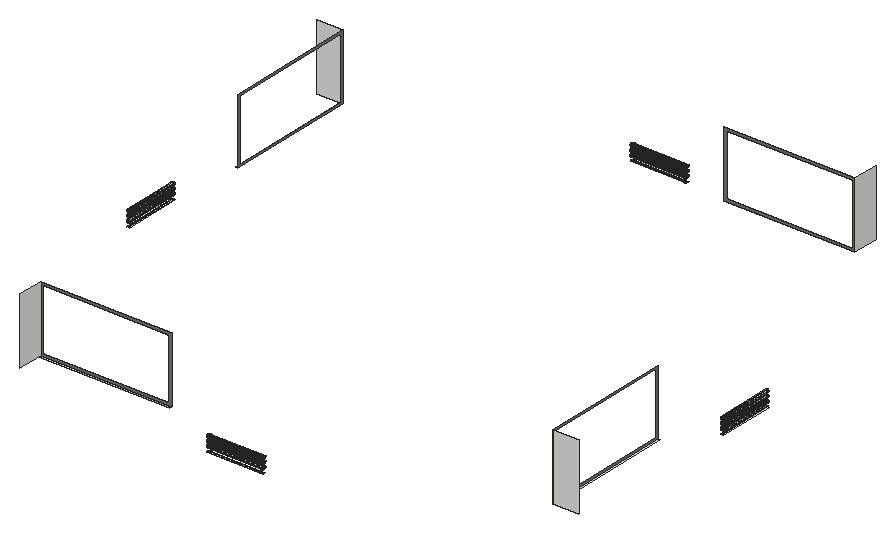
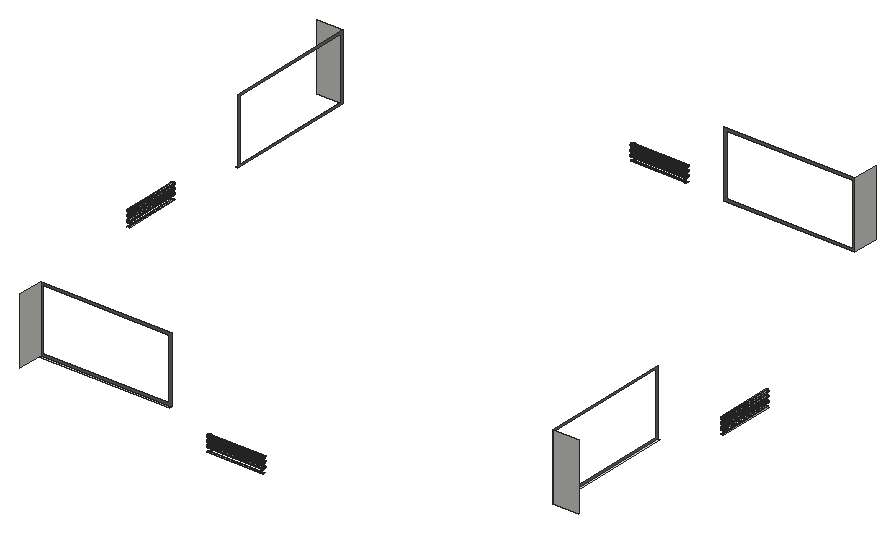
# SketchUp Ruby script. Lengths in inches.
U = 1.inch
M = Sketchup.active_model
def pt(a) = Geom::Point3d.new(a.map { |v| v * U })
def face(e, loops, mat)
  f = e.add_face(loops[0].map { |a| pt(a) })
  loops[1..].each { |l| e.add_face(l.map { |a| pt(a) }).erase! }
  f.material = f.back_material = mat if mat
  f
end
# faces: each face lists its corners as indices into pts; further lists are holes
def faces(e, pts, list, mat = nil) = list.each { |f| face(e, (f[0].is_a?(Array) ? f : [f]).map { |l| l.map { |i| pts[i] } }, mat) }
# xy, xz, yz: faces in a plane at the given z, y or x. An outline is a flat list of corners, or four numbers for a rectangle; further outlines are holes
def ring(l) = l.size == 4 ? [[l[0], l[1]], [l[2], l[1]], [l[2], l[3]], [l[0], l[3]]] : l.each_slice(2).to_a
def flat(e, list, mat, &to3) = list.each { |f| face(e, (f[0].is_a?(Array) ? f : [f]).map { |l| ring(l).map { |u, v| to3.(u, v) } }, mat) }
def xy(e, z, list, mat = nil) = flat(e, list, mat) { |x, y| [x, y, z] }
def xz(e, y, list, mat = nil) = flat(e, list, mat) { |x, z| [x, y, z] }
def yz(e, x, list, mat = nil) = flat(e, list, mat) { |y, z| [x, y, z] }
def lines(e, pts, list) = list.each { |a, b| e.add_line(pt(pts[a]), pt(pts[b])) }
# prism: a flat outline (further loops are holes) pulled along v
def prism(e, loops, v, mat = nil)
  f = face(e, loops, mat); d = Geom::Vector3d.new(v.map { |x| x * U })
  f.pushpull(f.normal.samedirection?(d) ? d.length : -d.length)
end
def box(e, o, s, mat = nil) = prism(e, [[o, [o[0] + s[0], o[1], o[2]], [o[0] + s[0], o[1] + s[1], o[2]], [o[0], o[1] + s[1], o[2]]]], [0, 0, s[2]], mat)
def at(x, y, z, deg = 0) = Geom::Transformation.translation(pt([x, y, z])) * Geom::Transformation.rotation(ORIGIN, Z_AXIS, deg.degrees)
def axes(o, x, y, z) = Geom::Transformation.new([*x, 0, *y, 0, *z, 0, *pt(o).to_a, 1])
def part(name) = M.definitions.add(name)
# library, detail: a bought-in or finely detailed component or shape, given as its bounding box
def library(name, o, s) = part(name).tap { |d| box(d.entities, o, s) }
def detail(e, o, s) = box(e.add_group.entities, o, s)
def put(e, d, t, mat = nil) = e.add_instance(d, t).tap { |i| i.material = mat if mat }
def group(e, t, mat = nil) = e.add_group.tap { |g| g.transformation = t; g.material = mat if mat }.entities
root = M.entities
M.materials.add("[Metal Seamed]").color = [118, 119, 115]
xy(root,893.76,[[306.65,96.8125,641.22,102.8125],[1482,271.47,1488,606.03],[132,943.59,138,1278.16],[978.78,1446.8125,1313.35,1452.8125]])
xz(root,102.8125,[[[306.65,893.76,641.22,1062.625],[312.65,899.76,635.22,1056.625]]],"[Metal Seamed]")
xz(root,271.47,[[1482,893.76,1548,1062.625]])
xz(root,1278.16,[[72,893.76,138,1062.625]])
xz(root,1446.8125,[[[978.78,893.76,1313.35,1062.625],[984.78,899.76,1307.35,1056.625]]],"[Metal Seamed]")
yz(root,138,[[[943.59,893.76,1278.16,1062.625],[949.59,899.76,1272.16,1056.625]]],"[Metal Seamed]")
yz(root,306.65,[[36.8125,893.76,102.8125,1062.625]])
yz(root,1313.35,[[1446.8125,893.76,1512.8125,1062.625]])
yz(root,1482,[[[271.47,893.76,606.03,1062.625],[277.47,899.76,600.03,1056.625]]],"[Metal Seamed]")
p = [[922.01,45.15,863.55],[922.01,45.73,864.3125],[778.64,45.73,864.3125],[778.64,45.15,863.55],[922.01,50.95,864.3125],[922.01,51.53,863.55],
  [778.64,51.53,863.55],[778.64,50.95,864.3125],[80.33,662.8,863.55],[80.92,662.8,864.3125],[80.92,806.17,864.3125],[80.33,806.17,863.55],
  [86.13,662.8,864.3125],[86.72,662.8,863.55],[86.72,806.17,863.55],[86.13,806.17,864.3125],[1533.87,886.83,864.3125],[1533.28,886.83,863.55],
  [1533.28,743.45,863.55],[1533.87,743.45,864.3125],[1539.67,886.83,863.55],[1539.08,886.83,864.3125],[1539.08,743.45,864.3125],[1539.67,743.45,863.55],
  [697.99,1498.68,864.3125],[697.99,1498.09,863.55],[841.36,1498.09,863.55],[841.36,1498.68,864.3125],[697.99,1504.48,863.55],[697.99,1503.89,864.3125],
  [841.36,1503.89,864.3125],[841.36,1504.48,863.55],[922.01,46.5,864.9],[778.64,46.5,864.9],[922.01,50.18,864.9],[778.64,50.18,864.9],
  [81.68,662.8,864.9],[81.68,806.17,864.9],[85.37,662.8,864.9],[85.37,806.17,864.9],[1534.63,886.83,864.9],[1534.63,743.45,864.9],
  [1538.32,886.83,864.9],[1538.32,743.45,864.9],[697.99,1499.44,864.9],[841.36,1499.44,864.9],[697.99,1503.13,864.9],[841.36,1503.13,864.9],
  [922.01,47.38,865.27],[778.64,47.38,865.27],[922.01,49.29,865.27],[778.64,49.29,865.27],[82.57,662.8,865.27],[82.57,806.17,865.27],
  [84.48,662.8,865.27],[84.48,806.17,865.27],[1535.52,886.83,865.27],[1535.52,743.45,865.27],[1537.43,886.83,865.27],[1537.43,743.45,865.27],
  [697.99,1500.33,865.27],[841.36,1500.33,865.27],[697.99,1502.24,865.27],[841.36,1502.24,865.27],[922.01,48.34,865.39],[778.64,48.34,865.39],
  [83.53,662.8,865.39],[83.53,806.17,865.39],[1536.47,886.83,865.39],[1536.47,743.45,865.39],[697.99,1501.28,865.39],[841.36,1501.28,865.39],
  [922.01,48.34,873.02],[922.01,47.38,873.14],[778.64,47.38,873.14],[778.64,48.34,873.02],[922.01,49.29,873.14],[778.64,49.29,873.14],
  [83.53,662.8,873.02],[82.57,662.8,873.14],[82.57,806.17,873.14],[83.53,806.17,873.02],[84.48,662.8,873.14],[84.48,806.17,873.14],
  [1535.52,886.83,873.14],[1536.47,886.83,873.02],[1536.47,743.45,873.02],[1535.52,743.45,873.14],[1537.43,886.83,873.14],[1537.43,743.45,873.14],
  [697.99,1500.33,873.14],[697.99,1501.28,873.02],[841.36,1501.28,873.02],[841.36,1500.33,873.14],[697.99,1502.24,873.14],[841.36,1502.24,873.14],
  [922.01,46.5,873.51],[778.64,46.5,873.51],[922.01,50.18,873.51],[778.64,50.18,873.51],[81.68,662.8,873.51],[81.68,806.17,873.51],
  [85.37,662.8,873.51],[85.37,806.17,873.51],[1534.63,886.83,873.51],[1534.63,743.45,873.51],[1538.32,886.83,873.51],[1538.32,743.45,873.51],
  [697.99,1499.44,873.51],[841.36,1499.44,873.51],[697.99,1503.13,873.51],[841.36,1503.13,873.51],[922.01,45.73,874.1],[778.64,45.73,874.1],
  [922.01,50.95,874.1],[778.64,50.95,874.1],[80.92,662.8,874.1],[80.92,806.17,874.1],[86.13,662.8,874.1],[86.13,806.17,874.1],
  [1533.87,886.83,874.1],[1533.87,743.45,874.1],[1539.08,886.83,874.1],[1539.08,743.45,874.1],[697.99,1498.68,874.1],[841.36,1498.68,874.1],
  [697.99,1503.89,874.1],[841.36,1503.89,874.1],[922.01,45.15,874.86],[778.64,45.15,874.86],[922.01,51.53,874.86],[778.64,51.53,874.86],
  [80.33,662.8,874.86],[80.33,806.17,874.86],[86.72,662.8,874.86],[86.72,806.17,874.86],[1533.28,886.83,874.86],[1533.28,743.45,874.86],
  [1539.67,886.83,874.86],[1539.67,743.45,874.86],[697.99,1498.09,874.86],[841.36,1498.09,874.86],[697.99,1504.48,874.86],[841.36,1504.48,874.86],
  [922.01,44.78,875.75],[778.64,44.78,875.75],[922.01,51.9,875.75],[778.64,51.9,875.75],[79.97,662.8,875.75],[79.97,806.17,875.75],
  [87.09,662.8,875.75],[87.09,806.17,875.75],[1532.91,886.83,875.75],[1532.91,743.45,875.75],[1540.03,886.83,875.75],[1540.03,743.45,875.75],
  [697.99,1497.72,875.75],[841.36,1497.72,875.75],[697.99,1504.85,875.75],[841.36,1504.85,875.75],[922.01,44.65,876.7],[778.64,44.65,876.7],
  [922.01,52.03,876.7],[778.64,52.03,876.7],[79.84,662.8,876.7],[79.84,806.17,876.7],[87.21,662.8,876.7],[87.21,806.17,876.7],
  [1532.79,886.83,876.7],[1532.79,743.45,876.7],[1540.16,886.83,876.7],[1540.16,743.45,876.7],[697.99,1497.6,876.7],[841.36,1497.6,876.7],
  [697.99,1504.97,876.7],[841.36,1504.97,876.7],[922.01,44.78,877.66],[778.64,44.78,877.66],[922.01,51.9,877.66],[778.64,51.9,877.66],
  [79.97,662.8,877.66],[79.97,806.17,877.66],[87.09,662.8,877.66],[87.09,806.17,877.66],[1532.91,886.83,877.66],[1532.91,743.45,877.66],
  [1540.03,886.83,877.66],[1540.03,743.45,877.66],[697.99,1497.72,877.66],[841.36,1497.72,877.66],[697.99,1504.85,877.66],[841.36,1504.85,877.66],
  [922.01,45.15,878.55],[778.64,45.15,878.55],[922.01,51.53,878.55],[778.64,51.53,878.55],[80.33,662.8,878.55],[80.33,806.17,878.55],
  [86.72,662.8,878.55],[86.72,806.17,878.55],[1533.28,886.83,878.55],[1533.28,743.45,878.55],[1539.67,886.83,878.55],[1539.67,743.45,878.55],
  [697.99,1498.09,878.55],[841.36,1498.09,878.55],[697.99,1504.48,878.55],[841.36,1504.48,878.55],[922.01,45.73,879.3125],[778.64,45.73,879.3125],
  [922.01,50.95,879.3125],[778.64,50.95,879.3125],[80.92,662.8,879.3125],[80.92,806.17,879.3125],[86.13,662.8,879.3125],[86.13,806.17,879.3125],
  [1533.87,886.83,879.3125],[1533.87,743.45,879.3125],[1539.08,886.83,879.3125],[1539.08,743.45,879.3125],[697.99,1498.68,879.3125],[841.36,1498.68,879.3125],
  [697.99,1503.89,879.3125],[841.36,1503.89,879.3125],[922.01,46.5,879.9],[778.64,46.5,879.9],[922.01,50.18,879.9],[778.64,50.18,879.9],
  [81.68,662.8,879.9],[81.68,806.17,879.9],[85.37,662.8,879.9],[85.37,806.17,879.9],[1534.63,886.83,879.9],[1534.63,743.45,879.9],
  [1538.32,886.83,879.9],[1538.32,743.45,879.9],[697.99,1499.44,879.9],[841.36,1499.44,879.9],[697.99,1503.13,879.9],[841.36,1503.13,879.9],
  [922.01,47.38,880.27],[778.64,47.38,880.27],[922.01,49.29,880.27],[778.64,49.29,880.27],[82.57,662.8,880.27],[82.57,806.17,880.27],
  [84.48,662.8,880.27],[84.48,806.17,880.27],[1535.52,886.83,880.27],[1535.52,743.45,880.27],[1537.43,886.83,880.27],[1537.43,743.45,880.27],
  [697.99,1500.33,880.27],[841.36,1500.33,880.27],[697.99,1502.24,880.27],[841.36,1502.24,880.27],[922.01,48.34,880.39],[778.64,48.34,880.39],
  [83.53,662.8,880.39],[83.53,806.17,880.39],[1536.47,886.83,880.39],[1536.47,743.45,880.39],[697.99,1501.28,880.39],[841.36,1501.28,880.39],
  [922.01,48.34,885.02],[922.01,47.38,885.14],[778.64,47.38,885.14],[778.64,48.34,885.02],[922.01,49.29,885.14],[778.64,49.29,885.14],
  [83.53,662.8,885.02],[82.57,662.8,885.14],[82.57,806.17,885.14],[83.53,806.17,885.02],[84.48,662.8,885.14],[84.48,806.17,885.14],
  [1535.52,886.83,885.14],[1536.47,886.83,885.02],[1536.47,743.45,885.02],[1535.52,743.45,885.14],[1537.43,886.83,885.14],[1537.43,743.45,885.14],
  [697.99,1500.33,885.14],[697.99,1501.28,885.02],[841.36,1501.28,885.02],[841.36,1500.33,885.14],[697.99,1502.24,885.14],[841.36,1502.24,885.14],
  [922.01,46.5,885.51],[778.64,46.5,885.51],[922.01,50.18,885.51],[778.64,50.18,885.51],[81.68,662.8,885.51],[81.68,806.17,885.51],
  [85.37,662.8,885.51],[85.37,806.17,885.51],[1534.63,886.83,885.51],[1534.63,743.45,885.51],[1538.32,886.83,885.51],[1538.32,743.45,885.51],
  [697.99,1499.44,885.51],[841.36,1499.44,885.51],[697.99,1503.13,885.51],[841.36,1503.13,885.51],[922.01,45.73,886.1],[778.64,45.73,886.1],
  [922.01,50.95,886.1],[778.64,50.95,886.1],[80.92,662.8,886.1],[80.92,806.17,886.1],[86.13,662.8,886.1],[86.13,806.17,886.1],
  [1533.87,886.83,886.1],[1533.87,743.45,886.1],[1539.08,886.83,886.1],[1539.08,743.45,886.1],[697.99,1498.68,886.1],[841.36,1498.68,886.1],
  [697.99,1503.89,886.1],[841.36,1503.89,886.1],[922.01,45.15,886.86],[778.64,45.15,886.86],[922.01,51.53,886.86],[778.64,51.53,886.86],
  [80.33,662.8,886.86],[80.33,806.17,886.86],[86.72,662.8,886.86],[86.72,806.17,886.86],[1533.28,886.83,886.86],[1533.28,743.45,886.86],
  [1539.67,886.83,886.86],[1539.67,743.45,886.86],[697.99,1498.09,886.86],[841.36,1498.09,886.86],[697.99,1504.48,886.86],[841.36,1504.48,886.86],
  [922.01,44.78,887.75],[778.64,44.78,887.75],[922.01,51.9,887.75],[778.64,51.9,887.75],[79.97,662.8,887.75],[79.97,806.17,887.75],
  [87.09,662.8,887.75],[87.09,806.17,887.75],[1532.91,886.83,887.75],[1532.91,743.45,887.75],[1540.03,886.83,887.75],[1540.03,743.45,887.75],
  [697.99,1497.72,887.75],[841.36,1497.72,887.75],[697.99,1504.85,887.75],[841.36,1504.85,887.75],[922.01,44.65,888.7],[778.64,44.65,888.7],
  [922.01,52.03,888.7],[778.64,52.03,888.7],[79.84,662.8,888.7],[79.84,806.17,888.7],[87.21,662.8,888.7],[87.21,806.17,888.7],
  [1532.79,886.83,888.7],[1532.79,743.45,888.7],[1540.16,886.83,888.7],[1540.16,743.45,888.7],[697.99,1497.6,888.7],[841.36,1497.6,888.7],
  [697.99,1504.97,888.7],[841.36,1504.97,888.7],[922.01,44.78,889.66],[778.64,44.78,889.66],[922.01,51.9,889.66],[778.64,51.9,889.66],
  [79.97,662.8,889.66],[79.97,806.17,889.66],[87.09,662.8,889.66],[87.09,806.17,889.66],[1532.91,886.83,889.66],[1532.91,743.45,889.66],
  [1540.03,886.83,889.66],[1540.03,743.45,889.66],[697.99,1497.72,889.66],[841.36,1497.72,889.66],[697.99,1504.85,889.66],[841.36,1504.85,889.66],
  [922.01,45.15,890.55],[778.64,45.15,890.55],[922.01,51.53,890.55],[778.64,51.53,890.55],[80.33,662.8,890.55],[80.33,806.17,890.55],
  [86.72,662.8,890.55],[86.72,806.17,890.55],[1533.28,886.83,890.55],[1533.28,743.45,890.55],[1539.67,886.83,890.55],[1539.67,743.45,890.55],
  [697.99,1498.09,890.55],[841.36,1498.09,890.55],[697.99,1504.48,890.55],[841.36,1504.48,890.55],[922.01,45.73,891.3125],[778.64,45.73,891.3125],
  [922.01,50.95,891.3125],[778.64,50.95,891.3125],[80.92,662.8,891.3125],[80.92,806.17,891.3125],[86.13,662.8,891.3125],[86.13,806.17,891.3125],
  [1533.87,886.83,891.3125],[1533.87,743.45,891.3125],[1539.08,886.83,891.3125],[1539.08,743.45,891.3125],[697.99,1498.68,891.3125],[841.36,1498.68,891.3125],
  [697.99,1503.89,891.3125],[841.36,1503.89,891.3125],[922.01,46.5,891.9],[778.64,46.5,891.9],[922.01,50.18,891.9],[778.64,50.18,891.9],
  [81.68,662.8,891.9],[81.68,806.17,891.9],[85.37,662.8,891.9],[85.37,806.17,891.9],[1534.63,886.83,891.9],[1534.63,743.45,891.9],
  [1538.32,886.83,891.9],[1538.32,743.45,891.9],[697.99,1499.44,891.9],[841.36,1499.44,891.9],[697.99,1503.13,891.9],[841.36,1503.13,891.9],
  [922.01,47.38,892.27],[778.64,47.38,892.27],[922.01,49.29,892.27],[778.64,49.29,892.27],[82.57,662.8,892.27],[82.57,806.17,892.27],
  [84.48,662.8,892.27],[84.48,806.17,892.27],[1535.52,886.83,892.27],[1535.52,743.45,892.27],[1537.43,886.83,892.27],[1537.43,743.45,892.27],
  [697.99,1500.33,892.27],[841.36,1500.33,892.27],[697.99,1502.24,892.27],[841.36,1502.24,892.27],[922.01,48.34,892.39],[778.64,48.34,892.39],
  [83.53,662.8,892.39],[83.53,806.17,892.39],[1536.47,886.83,892.39],[1536.47,743.45,892.39],[697.99,1501.28,892.39],[841.36,1501.28,892.39],
  [922.01,48.34,897.02],[922.01,47.38,897.14],[778.64,47.38,897.14],[778.64,48.34,897.02],[922.01,49.29,897.14],[778.64,49.29,897.14],
  [83.53,662.8,897.02],[82.57,662.8,897.14],[82.57,806.17,897.14],[83.53,806.17,897.02],[84.48,662.8,897.14],[84.48,806.17,897.14],
  [1535.52,886.83,897.14],[1536.47,886.83,897.02],[1536.47,743.45,897.02],[1535.52,743.45,897.14],[1537.43,886.83,897.14],[1537.43,743.45,897.14],
  [697.99,1500.33,897.14],[697.99,1501.28,897.02],[841.36,1501.28,897.02],[841.36,1500.33,897.14],[697.99,1502.24,897.14],[841.36,1502.24,897.14],
  [922.01,46.5,897.51],[778.64,46.5,897.51],[922.01,50.18,897.51],[778.64,50.18,897.51],[81.68,662.8,897.51],[81.68,806.17,897.51],
  [85.37,662.8,897.51],[85.37,806.17,897.51],[1534.63,886.83,897.51],[1534.63,743.45,897.51],[1538.32,886.83,897.51],[1538.32,743.45,897.51],
  [697.99,1499.44,897.51],[841.36,1499.44,897.51],[697.99,1503.13,897.51],[841.36,1503.13,897.51],[922.01,45.73,898.1],[778.64,45.73,898.1],
  [922.01,50.95,898.1],[778.64,50.95,898.1],[80.92,662.8,898.1],[80.92,806.17,898.1],[86.13,662.8,898.1],[86.13,806.17,898.1],
  [1533.87,886.83,898.1],[1533.87,743.45,898.1],[1539.08,886.83,898.1],[1539.08,743.45,898.1],[697.99,1498.68,898.1],[841.36,1498.68,898.1],
  [697.99,1503.89,898.1],[841.36,1503.89,898.1],[922.01,45.15,898.86],[778.64,45.15,898.86],[922.01,51.53,898.86],[778.64,51.53,898.86],
  [80.33,662.8,898.86],[80.33,806.17,898.86],[86.72,662.8,898.86],[86.72,806.17,898.86],[1533.28,886.83,898.86],[1533.28,743.45,898.86],
  [1539.67,886.83,898.86],[1539.67,743.45,898.86],[697.99,1498.09,898.86],[841.36,1498.09,898.86],[697.99,1504.48,898.86],[841.36,1504.48,898.86],
  [922.01,44.78,899.75],[778.64,44.78,899.75],[922.01,51.9,899.75],[778.64,51.9,899.75],[79.97,662.8,899.75],[79.97,806.17,899.75],
  [87.09,662.8,899.75],[87.09,806.17,899.75],[1532.91,886.83,899.75],[1532.91,743.45,899.75],[1540.03,886.83,899.75],[1540.03,743.45,899.75],
  [697.99,1497.72,899.75],[841.36,1497.72,899.75],[697.99,1504.85,899.75],[841.36,1504.85,899.75],[922.01,44.65,900.7],[778.64,44.65,900.7],
  [922.01,52.03,900.7],[778.64,52.03,900.7],[79.84,662.8,900.7],[79.84,806.17,900.7],[87.21,662.8,900.7],[87.21,806.17,900.7],
  [1532.79,886.83,900.7],[1532.79,743.45,900.7],[1540.16,886.83,900.7],[1540.16,743.45,900.7],[697.99,1497.6,900.7],[841.36,1497.6,900.7],
  [697.99,1504.97,900.7],[841.36,1504.97,900.7],[922.01,44.78,901.66],[778.64,44.78,901.66],[922.01,51.9,901.66],[778.64,51.9,901.66],
  [79.97,662.8,901.66],[79.97,806.17,901.66],[87.09,662.8,901.66],[87.09,806.17,901.66],[1532.91,886.83,901.66],[1532.91,743.45,901.66],
  [1540.03,886.83,901.66],[1540.03,743.45,901.66],[697.99,1497.72,901.66],[841.36,1497.72,901.66],[697.99,1504.85,901.66],[841.36,1504.85,901.66],
  [922.01,45.15,902.55],[778.64,45.15,902.55],[922.01,51.53,902.55],[778.64,51.53,902.55],[80.33,662.8,902.55],[80.33,806.17,902.55],
  [86.72,662.8,902.55],[86.72,806.17,902.55],[1533.28,886.83,902.55],[1533.28,743.45,902.55],[1539.67,886.83,902.55],[1539.67,743.45,902.55],
  [697.99,1498.09,902.55],[841.36,1498.09,902.55],[697.99,1504.48,902.55],[841.36,1504.48,902.55],[922.01,45.73,903.3125],[778.64,45.73,903.3125],
  [922.01,50.95,903.3125],[778.64,50.95,903.3125],[80.92,662.8,903.3125],[80.92,806.17,903.3125],[86.13,662.8,903.3125],[86.13,806.17,903.3125],
  [1533.87,886.83,903.3125],[1533.87,743.45,903.3125],[1539.08,886.83,903.3125],[1539.08,743.45,903.3125],[697.99,1498.68,903.3125],[841.36,1498.68,903.3125],
  [697.99,1503.89,903.3125],[841.36,1503.89,903.3125],[922.01,46.5,903.9],[778.64,46.5,903.9],[922.01,50.18,903.9],[778.64,50.18,903.9],
  [81.68,662.8,903.9],[81.68,806.17,903.9],[85.37,662.8,903.9],[85.37,806.17,903.9],[1534.63,886.83,903.9],[1534.63,743.45,903.9],
  [1538.32,886.83,903.9],[1538.32,743.45,903.9],[697.99,1499.44,903.9],[841.36,1499.44,903.9],[697.99,1503.13,903.9],[841.36,1503.13,903.9],
  [922.01,47.38,904.27],[778.64,47.38,904.27],[922.01,49.29,904.27],[778.64,49.29,904.27],[82.57,662.8,904.27],[82.57,806.17,904.27],
  [84.48,662.8,904.27],[84.48,806.17,904.27],[1535.52,886.83,904.27],[1535.52,743.45,904.27],[1537.43,886.83,904.27],[1537.43,743.45,904.27],
  [697.99,1500.33,904.27],[841.36,1500.33,904.27],[697.99,1502.24,904.27],[841.36,1502.24,904.27],[922.01,48.34,904.39],[778.64,48.34,904.39],
  [83.53,662.8,904.39],[83.53,806.17,904.39],[1536.47,886.83,904.39],[1536.47,743.45,904.39],[697.99,1501.28,904.39],[841.36,1501.28,904.39]]
faces(root,p,[[0,1,2,3],[4,5,6,7],[8,9,10,11],[12,13,14,15],[16,17,18,19],[20,21,22,23],[24,25,26,27],[28,29,30,31],
  [1,32,33,2],[34,4,7,35],[9,36,37,10],[38,12,15,39],[40,16,19,41],[21,42,43,22],[44,24,27,45],[29,46,47,30],
  [32,48,49,33],[50,34,35,51],[36,52,53,37],[54,38,39,55],[56,40,41,57],[42,58,59,43],[60,44,45,61],[46,62,63,47],
  [48,64,65,49],[64,50,51,65],[52,66,67,53],[66,54,55,67],[68,56,57,69],[58,68,69,59],[70,60,61,71],[62,70,71,63],
  [72,73,74,75],[76,72,75,77],[78,79,80,81],[82,78,81,83],[84,85,86,87],[85,88,89,86],[90,91,92,93],[91,94,95,92],
  [73,96,97,74],[98,76,77,99],[79,100,101,80],[102,82,83,103],[104,84,87,105],[88,106,107,89],[108,90,93,109],[94,110,111,95],
  [96,112,113,97],[114,98,99,115],[100,116,117,101],[118,102,103,119],[120,104,105,121],[106,122,123,107],[124,108,109,125],[110,126,127,111],
  [112,128,129,113],[130,114,115,131],[116,132,133,117],[134,118,119,135],[136,120,121,137],[122,138,139,123],[140,124,125,141],[126,142,143,127],
  [128,144,145,129],[146,130,131,147],[132,148,149,133],[150,134,135,151],[152,136,137,153],[138,154,155,139],[156,140,141,157],[142,158,159,143],
  [144,160,161,145],[162,146,147,163],[148,164,165,149],[166,150,151,167],[168,152,153,169],[154,170,171,155],[172,156,157,173],[158,174,175,159],
  [160,176,177,161],[178,162,163,179],[164,180,181,165],[182,166,167,183],[184,168,169,185],[170,186,187,171],[188,172,173,189],[174,190,191,175],
  [176,192,193,177],[194,178,179,195],[180,196,197,181],[198,182,183,199],[200,184,185,201],[186,202,203,187],[204,188,189,205],[190,206,207,191],
  [192,208,209,193],[210,194,195,211],[196,212,213,197],[214,198,199,215],[216,200,201,217],[202,218,219,203],[220,204,205,221],[206,222,223,207],
  [208,224,225,209],[226,210,211,227],[212,228,229,213],[230,214,215,231],[232,216,217,233],[218,234,235,219],[236,220,221,237],[222,238,239,223],
  [224,240,241,225],[242,226,227,243],[228,244,245,229],[246,230,231,247],[248,232,233,249],[234,250,251,235],[252,236,237,253],[238,254,255,239],
  [240,256,257,241],[256,242,243,257],[244,258,259,245],[258,246,247,259],[260,248,249,261],[250,260,261,251],[262,252,253,263],[254,262,263,255],
  [264,265,266,267],[268,264,267,269],[270,271,272,273],[274,270,273,275],[276,277,278,279],[277,280,281,278],[282,283,284,285],[283,286,287,284],
  [265,288,289,266],[290,268,269,291],[271,292,293,272],[294,274,275,295],[296,276,279,297],[280,298,299,281],[300,282,285,301],[286,302,303,287],
  [288,304,305,289],[306,290,291,307],[292,308,309,293],[310,294,295,311],[312,296,297,313],[298,314,315,299],[316,300,301,317],[302,318,319,303],
  [304,320,321,305],[322,306,307,323],[308,324,325,309],[326,310,311,327],[328,312,313,329],[314,330,331,315],[332,316,317,333],[318,334,335,319],
  [320,336,337,321],[338,322,323,339],[324,340,341,325],[342,326,327,343],[344,328,329,345],[330,346,347,331],[348,332,333,349],[334,350,351,335],
  [336,352,353,337],[354,338,339,355],[340,356,357,341],[358,342,343,359],[360,344,345,361],[346,362,363,347],[364,348,349,365],[350,366,367,351],
  [352,368,369,353],[370,354,355,371],[356,372,373,357],[374,358,359,375],[376,360,361,377],[362,378,379,363],[380,364,365,381],[366,382,383,367],
  [368,384,385,369],[386,370,371,387],[372,388,389,373],[390,374,375,391],[392,376,377,393],[378,394,395,379],[396,380,381,397],[382,398,399,383],
  [384,400,401,385],[402,386,387,403],[388,404,405,389],[406,390,391,407],[408,392,393,409],[394,410,411,395],[412,396,397,413],[398,414,415,399],
  [400,416,417,401],[418,402,403,419],[404,420,421,405],[422,406,407,423],[424,408,409,425],[410,426,427,411],[428,412,413,429],[414,430,431,415],
  [416,432,433,417],[434,418,419,435],[420,436,437,421],[438,422,423,439],[440,424,425,441],[426,442,443,427],[444,428,429,445],[430,446,447,431],
  [432,448,449,433],[448,434,435,449],[436,450,451,437],[450,438,439,451],[452,440,441,453],[442,452,453,443],[454,444,445,455],[446,454,455,447],
  [456,457,458,459],[460,456,459,461],[462,463,464,465],[466,462,465,467],[468,469,470,471],[469,472,473,470],[474,475,476,477],[475,478,479,476],
  [457,480,481,458],[482,460,461,483],[463,484,485,464],[486,466,467,487],[488,468,471,489],[472,490,491,473],[492,474,477,493],[478,494,495,479],
  [480,496,497,481],[498,482,483,499],[484,500,501,485],[502,486,487,503],[504,488,489,505],[490,506,507,491],[508,492,493,509],[494,510,511,495],
  [496,512,513,497],[514,498,499,515],[500,516,517,501],[518,502,503,519],[520,504,505,521],[506,522,523,507],[524,508,509,525],[510,526,527,511],
  [512,528,529,513],[530,514,515,531],[516,532,533,517],[534,518,519,535],[536,520,521,537],[522,538,539,523],[540,524,525,541],[526,542,543,527],
  [528,544,545,529],[546,530,531,547],[532,548,549,533],[550,534,535,551],[552,536,537,553],[538,554,555,539],[556,540,541,557],[542,558,559,543],
  [544,560,561,545],[562,546,547,563],[548,564,565,549],[566,550,551,567],[568,552,553,569],[554,570,571,555],[572,556,557,573],[558,574,575,559],
  [560,576,577,561],[578,562,563,579],[564,580,581,565],[582,566,567,583],[584,568,569,585],[570,586,587,571],[588,572,573,589],[574,590,591,575],
  [576,592,593,577],[594,578,579,595],[580,596,597,581],[598,582,583,599],[600,584,585,601],[586,602,603,587],[604,588,589,605],[590,606,607,591],
  [592,608,609,593],[610,594,595,611],[596,612,613,597],[614,598,599,615],[616,600,601,617],[602,618,619,603],[620,604,605,621],[606,622,623,607],
  [608,624,625,609],[626,610,611,627],[612,628,629,613],[630,614,615,631],[632,616,617,633],[618,634,635,619],[636,620,621,637],[622,638,639,623],
  [624,640,641,625],[640,626,627,641],[628,642,643,629],[642,630,631,643],[644,632,633,645],[634,644,645,635],[646,636,637,647],[638,646,647,639]])
